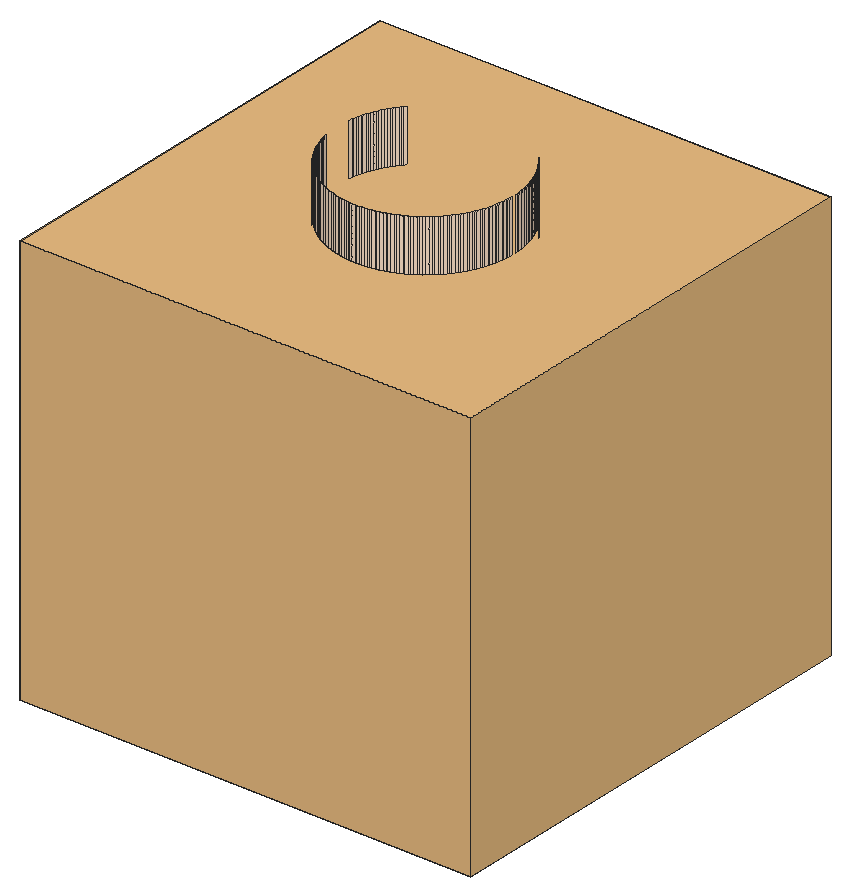
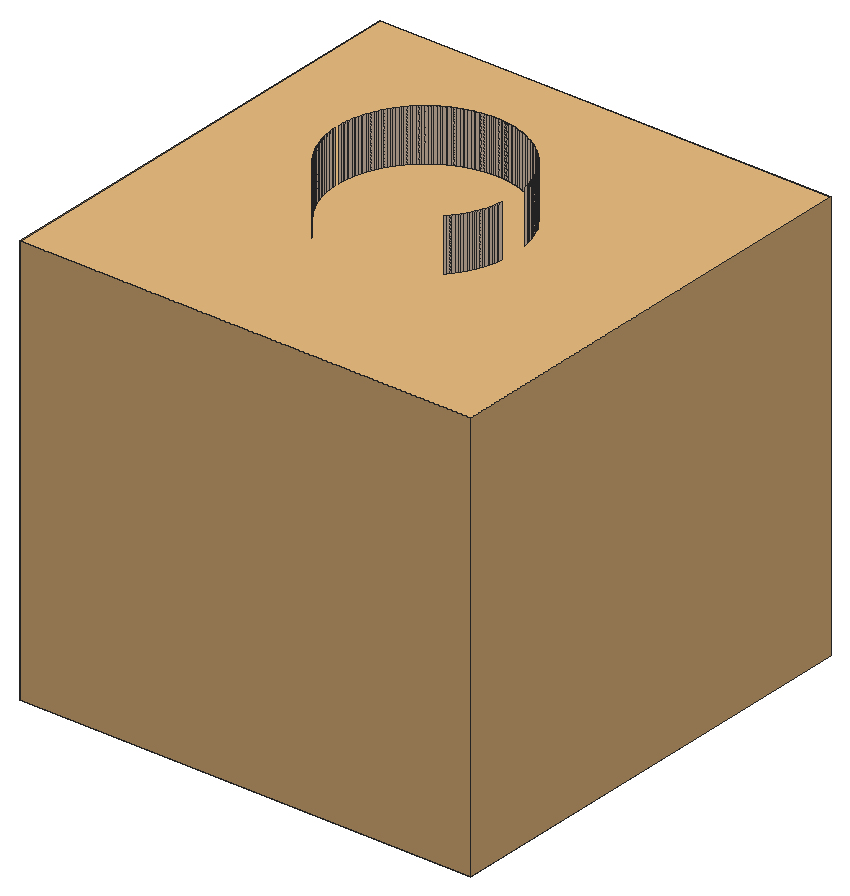
# SketchUp Ruby script. Lengths in inches.
U = 1.inch
M = Sketchup.active_model
def pt(a) = Geom::Point3d.new(a.map { |v| v * U })
def face(e, loops, mat)
  f = e.add_face(loops[0].map { |a| pt(a) })
  loops[1..].each { |l| e.add_face(l.map { |a| pt(a) }).erase! }
  f.material = f.back_material = mat if mat
  f
end
# faces: each face lists its corners as indices into pts; further lists are holes
def faces(e, pts, list, mat = nil) = list.each { |f| face(e, (f[0].is_a?(Array) ? f : [f]).map { |l| l.map { |i| pts[i] } }, mat) }
# xy, xz, yz: faces in a plane at the given z, y or x. An outline is a flat list of corners, or four numbers for a rectangle; further outlines are holes
def ring(l) = l.size == 4 ? [[l[0], l[1]], [l[2], l[1]], [l[2], l[3]], [l[0], l[3]]] : l.each_slice(2).to_a
def flat(e, list, mat, &to3) = list.each { |f| face(e, (f[0].is_a?(Array) ? f : [f]).map { |l| ring(l).map { |u, v| to3.(u, v) } }, mat) }
def xy(e, z, list, mat = nil) = flat(e, list, mat) { |x, y| [x, y, z] }
def xz(e, y, list, mat = nil) = flat(e, list, mat) { |x, z| [x, y, z] }
def yz(e, x, list, mat = nil) = flat(e, list, mat) { |y, z| [x, y, z] }
def lines(e, pts, list) = list.each { |a, b| e.add_line(pt(pts[a]), pt(pts[b])) }
# prism: a flat outline (further loops are holes) pulled along v
def prism(e, loops, v, mat = nil)
  f = face(e, loops, mat); d = Geom::Vector3d.new(v.map { |x| x * U })
  f.pushpull(f.normal.samedirection?(d) ? d.length : -d.length)
end
def box(e, o, s, mat = nil) = prism(e, [[o, [o[0] + s[0], o[1], o[2]], [o[0] + s[0], o[1] + s[1], o[2]], [o[0], o[1] + s[1], o[2]]]], [0, 0, s[2]], mat)
def at(x, y, z, deg = 0) = Geom::Transformation.translation(pt([x, y, z])) * Geom::Transformation.rotation(ORIGIN, Z_AXIS, deg.degrees)
def axes(o, x, y, z) = Geom::Transformation.new([*x, 0, *y, 0, *z, 0, *pt(o).to_a, 1])
def part(name) = M.definitions.add(name)
# library, detail: a bought-in or finely detailed component or shape, given as its bounding box
def library(name, o, s) = part(name).tap { |d| box(d.entities, o, s) }
def detail(e, o, s) = box(e.add_group.entities, o, s)
def put(e, d, t, mat = nil) = e.add_instance(d, t).tap { |i| i.material = mat if mat }
def group(e, t, mat = nil) = e.add_group.tap { |g| g.transformation = t; g.material = mat if mat }.entities
root = M.entities
M.materials.add("1122 AP 7994 PEACH ROSE").color = [254, 227, 201]
c1 = library("9",[-5.85,-5.85,-13.96],[15.28,15.28,13.96])
xz(root,174,[[52.82,278.82,52.9,281.82],[52.9,278.82,52.98,281.82],[52.98,278.82,53.06,281.82],[53.06,278.82,53.14,281.82]],"1122 AP 7994 PEACH ROSE")
yz(root,55.96,[[176.61,278.82,176.6875,281.82],[177.3125,278.82,177.39,281.82]],"1122 AP 7994 PEACH ROSE")
yz(root,55.98,[[176.84,278.82,176.92,281.82],[177.08,278.82,177.16,281.82]],"1122 AP 7994 PEACH ROSE")
p = [[52.51,174.04,278.82],[52.43,174.05,278.82],[52.43,174.05,281.82],[52.51,174.04,281.82],[52.59,174.03,278.82],[52.59,174.03,281.82],
  [52.67,174.02,278.82],[52.67,174.02,281.82],[52.75,174.01,278.82],[52.75,174.01,281.82],[52.82,174,278.82],[52.82,174,281.82],
  [53.22,174.01,278.82],[53.14,174,278.82],[53.14,174,281.82],[53.22,174.01,281.82],[53.29,174.02,278.82],[53.29,174.02,281.82],
  [53.37,174.03,278.82],[53.37,174.03,281.82],[53.45,174.04,278.82],[53.45,174.04,281.82],[53.53,174.05,278.82],[53.53,174.05,281.82],
  [52.05,174.15,278.82],[51.98,174.17,278.82],[51.98,174.17,281.82],[52.05,174.15,281.82],[52.13,174.125,278.82],[52.13,174.125,281.82],
  [52.2,174.1,278.82],[52.2,174.1,281.82],[52.28,174.08,278.82],[52.28,174.08,281.82],[52.36,174.07,278.82],[52.36,174.07,281.82],
  [53.6,174.07,278.82],[53.6,174.07,281.82],[53.68,174.08,278.82],[53.68,174.08,281.82],[53.76,174.1,278.82],[53.76,174.1,281.82],
  [53.83,174.125,278.82],[53.83,174.125,281.82],[53.91,174.15,278.82],[53.91,174.15,281.82],[53.98,174.17,278.82],[53.98,174.17,281.82],
  [51.83,174.23,278.82],[51.76,174.26,278.82],[51.76,174.26,281.82],[51.83,174.23,281.82],[51.91,174.2,278.82],[51.91,174.2,281.82],
  [54.06,174.2,278.82],[54.06,174.2,281.82],[54.13,174.23,278.82],[54.13,174.23,281.82],[54.2,174.26,278.82],[54.2,174.26,281.82],
  [51.62,174.33,278.82],[51.55,174.36,278.82],[51.55,174.36,281.82],[51.62,174.33,281.82],[51.6875,174.29,278.82],[51.6875,174.29,281.82],
  [54.27,174.29,278.82],[54.27,174.29,281.82],[54.34,174.33,278.82],[54.34,174.33,281.82],[54.41,174.36,278.82],[54.41,174.36,281.82],
  [51.41,174.44,278.82],[51.35,174.48,278.82],[51.35,174.48,281.82],[51.41,174.44,281.82],[51.48,174.4,278.82],[51.48,174.4,281.82],
  [54.48,174.4,278.82],[54.48,174.4,281.82],[54.55,174.44,278.82],[54.55,174.44,281.82],[54.61,174.48,278.82],[54.61,174.48,281.82],
  [51.28,174.53,278.82],[51.22,174.57,278.82],[51.22,174.57,281.82],[51.28,174.53,281.82],[54.68,174.53,278.82],[54.68,174.53,281.82],
  [54.74,174.57,278.82],[54.74,174.57,281.82],[51.15,174.62,278.82],[51.09,174.67,278.82],[51.09,174.67,281.82],[51.15,174.62,281.82],
  [54.81,174.62,278.82],[54.81,174.62,281.82],[54.87,174.67,278.82],[54.87,174.67,281.82],[51.03,174.72,278.82],[50.97,174.77,278.82],
  [50.97,174.77,281.82],[51.03,174.72,281.82],[54.93,174.72,278.82],[54.93,174.72,281.82],[54.99,174.77,278.82],[54.99,174.77,281.82],
  [50.92,174.82,278.82],[50.86,174.88,278.82],[50.86,174.88,281.82],[50.92,174.82,281.82],[55.05,174.82,278.82],[55.05,174.82,281.82],
  [55.1,174.88,278.82],[55.1,174.88,281.82],[50.8,174.93,278.82],[50.75,174.99,278.82],[50.75,174.99,281.82],[50.8,174.93,281.82],
  [55.16,174.93,278.82],[55.16,174.93,281.82],[55.21,174.99,278.82],[55.21,174.99,281.82],[50.7,175.05,278.82],[50.7,175.05,281.82],
  [55.26,175.05,278.82],[55.26,175.05,281.82],[50.65,175.11,278.82],[50.6,175.17,278.82],[50.6,175.17,281.82],[50.65,175.11,281.82],
  [55.3125,175.11,278.82],[55.3125,175.11,281.82],[55.36,175.17,278.82],[55.36,175.17,281.82],[50.55,175.24,278.82],[50.51,175.3,278.82],
  [50.51,175.3,281.82],[50.55,175.24,281.82],[55.41,175.24,278.82],[55.41,175.24,281.82],[55.45,175.3,278.82],[55.45,175.3,281.82],
  [50.46,175.37,278.82],[50.46,175.37,281.82],[55.5,175.37,278.82],[55.5,175.37,281.82],[50.42,175.43,278.82],[50.38,175.5,278.82],
  [50.38,175.5,281.82],[50.42,175.43,281.82],[55.54,175.43,278.82],[55.54,175.43,281.82],[55.58,175.5,278.82],[55.58,175.5,281.82],
  [50.34,175.57,278.82],[50.34,175.57,281.82],[55.62,175.57,278.82],[55.62,175.57,281.82],[50.31,175.64,278.82],[50.27,175.71,278.82],
  [50.27,175.71,281.82],[50.31,175.64,281.82],[55.65,175.64,278.82],[55.65,175.64,281.82],[55.6875,175.71,278.82],[55.6875,175.71,281.82],
  [50.24,175.78,278.82],[50.24,175.78,281.82],[55.72,175.78,278.82],[55.72,175.78,281.82],[50.21,175.85,278.82],[50.21,175.85,281.82],
  [55.75,175.85,278.82],[55.75,175.85,281.82],[50.18,175.92,278.82],[50.15,176,278.82],[50.15,176,281.82],[50.18,175.92,281.82],
  [55.78,175.92,278.82],[55.78,175.92,281.82],[55.81,176,278.82],[55.81,176,281.82],[50.13,176.07,278.82],[50.13,176.07,281.82],
  [55.83,176.07,278.82],[55.83,176.07,281.82],[50.1,176.15,278.82],[50.08,176.22,278.82],[50.08,176.22,281.82],[50.1,176.15,281.82],
  [55.86,176.15,278.82],[55.86,176.15,281.82],[55.88,176.22,278.82],[55.88,176.22,281.82],[50.0625,176.3,278.82],[50.0625,176.3,281.82],
  [55.9,176.3,278.82],[55.9,176.3,281.82],[50.05,176.375,278.82],[50.05,176.375,281.82],[55.92,176.375,278.82],[55.92,176.375,281.82],
  [50.03,176.45,278.82],[50.03,176.45,281.82],[55.93,176.45,278.82],[55.93,176.45,281.82],[55.94,176.53,278.82],[55.94,176.53,281.82],
  [55.96,176.61,278.82],[55.96,176.61,281.82],[55.97,176.76,278.82],[55.96,176.6875,278.82],[55.96,176.6875,281.82],[55.97,176.76,281.82],
  [55.98,176.84,278.82],[55.98,176.84,281.82],[55.96,177.3125,278.82],[55.97,177.24,278.82],[55.97,177.24,281.82],[55.96,177.3125,281.82],
  [55.98,177.16,278.82],[55.98,177.16,281.82],[55.94,177.47,278.82],[55.96,177.39,278.82],[55.96,177.39,281.82],[55.94,177.47,281.82],
  [50.02,177.47,278.82],[50.03,177.55,278.82],[50.03,177.55,281.82],[50.02,177.47,281.82],[50.05,177.625,278.82],[50.05,177.625,281.82],
  [55.92,177.625,278.82],[55.93,177.55,278.82],[55.93,177.55,281.82],[55.92,177.625,281.82],[50.0625,177.7,278.82],[50.0625,177.7,281.82],
  [55.9,177.7,278.82],[55.9,177.7,281.82],[50.08,177.78,278.82],[50.08,177.78,281.82],[55.88,177.78,278.82],[55.88,177.78,281.82],
  [50.1,177.85,278.82],[50.1,177.85,281.82],[55.86,177.85,278.82],[55.86,177.85,281.82],[50.13,177.93,278.82],[50.13,177.93,281.82],
  [50.15,178,278.82],[50.15,178,281.82],[55.81,178,278.82],[55.83,177.93,278.82],[55.83,177.93,281.82],[55.81,178,281.82],
  [50.18,178.08,278.82],[50.18,178.08,281.82],[55.78,178.08,278.82],[55.78,178.08,281.82],[50.21,178.15,278.82],[50.21,178.15,281.82],
  [50.24,178.22,278.82],[50.24,178.22,281.82],[55.72,178.22,278.82],[55.75,178.15,278.82],[55.75,178.15,281.82],[55.72,178.22,281.82],
  [50.27,178.29,278.82],[50.27,178.29,281.82],[55.6875,178.29,278.82],[55.6875,178.29,281.82],[50.31,178.36,278.82],[50.31,178.36,281.82],
  [55.65,178.36,278.82],[55.65,178.36,281.82],[50.34,178.43,278.82],[50.34,178.43,281.82],[50.38,178.5,278.82],[50.38,178.5,281.82],
  [55.58,178.5,278.82],[55.62,178.43,278.82],[55.62,178.43,281.82],[55.58,178.5,281.82],[50.42,178.57,278.82],[50.42,178.57,281.82],
  [55.54,178.57,278.82],[55.54,178.57,281.82],[50.46,178.63,278.82],[50.46,178.63,281.82],[50.51,178.7,278.82],[50.51,178.7,281.82],
  [55.45,178.7,278.82],[55.5,178.63,278.82],[55.5,178.63,281.82],[55.45,178.7,281.82],[50.55,178.76,278.82],[50.55,178.76,281.82],
  [55.41,178.76,278.82],[55.41,178.76,281.82],[50.6,178.83,278.82],[50.6,178.83,281.82],[50.65,178.89,278.82],[50.65,178.89,281.82],
  [55.3125,178.89,278.82],[55.36,178.83,278.82],[55.36,178.83,281.82],[55.3125,178.89,281.82],[50.7,178.95,278.82],[50.7,178.95,281.82],
  [50.75,179.01,278.82],[50.75,179.01,281.82],[55.21,179.01,278.82],[55.26,178.95,278.82],[55.26,178.95,281.82],[55.21,179.01,281.82]]
faces(root,p,[[0,1,2,3],[4,0,3,5],[6,4,5,7],[8,6,7,9],[10,8,9,11],[12,13,14,15],[16,12,15,17],[18,16,17,19],
  [20,18,19,21],[22,20,21,23],[24,25,26,27],[28,24,27,29],[30,28,29,31],[32,30,31,33],[34,32,33,35],[1,34,35,2],
  [36,22,23,37],[38,36,37,39],[40,38,39,41],[42,40,41,43],[44,42,43,45],[46,44,45,47],[48,49,50,51],[52,48,51,53],
  [25,52,53,26],[54,46,47,55],[56,54,55,57],[58,56,57,59],[60,61,62,63],[64,60,63,65],[49,64,65,50],[66,58,59,67],
  [68,66,67,69],[70,68,69,71],[72,73,74,75],[76,72,75,77],[61,76,77,62],[78,70,71,79],[80,78,79,81],[82,80,81,83],
  [84,85,86,87],[73,84,87,74],[88,82,83,89],[90,88,89,91],[92,93,94,95],[85,92,95,86],[96,90,91,97],[98,96,97,99],
  [100,101,102,103],[93,100,103,94],[104,98,99,105],[106,104,105,107],[108,109,110,111],[101,108,111,102],[112,106,107,113],[114,112,113,115],
  [116,117,118,119],[109,116,119,110],[120,114,115,121],[122,120,121,123],[117,124,125,118],[126,122,123,127],[128,129,130,131],[124,128,131,125],
  [132,126,127,133],[134,132,133,135],[136,137,138,139],[129,136,139,130],[140,134,135,141],[142,140,141,143],[137,144,145,138],[146,142,143,147],
  [148,149,150,151],[144,148,151,145],[152,146,147,153],[154,152,153,155],[149,156,157,150],[158,154,155,159],[160,161,162,163],[156,160,163,157],
  [164,158,159,165],[166,164,165,167],[161,168,169,162],[170,166,167,171],[168,172,173,169],[174,170,171,175],[176,177,178,179],[172,176,179,173],
  [180,174,175,181],[182,180,181,183],[177,184,185,178],[186,182,183,187],[188,189,190,191],[184,188,191,185],[192,186,187,193],[194,192,193,195],
  [189,196,197,190],[198,194,195,199],[196,200,201,197],[202,198,199,203],[200,204,205,201],[206,202,203,207],[208,206,207,209],[210,208,209,211],
  [212,213,214,215],[216,212,215,217],[218,219,220,221],[219,222,223,220],[224,225,226,227],[228,229,230,231],[229,232,233,230],[234,235,236,237],
  [235,224,227,236],[232,238,239,233],[240,234,237,241],[238,242,243,239],[244,240,241,245],[242,246,247,243],[248,244,245,249],[246,250,251,247],
  [250,252,253,251],[254,255,256,257],[255,248,249,256],[252,258,259,253],[260,254,257,261],[258,262,263,259],[262,264,265,263],[266,267,268,269],
  [267,260,261,268],[264,270,271,265],[272,266,269,273],[270,274,275,271],[276,272,273,277],[274,278,279,275],[278,280,281,279],[282,283,284,285],
  [283,276,277,284],[280,286,287,281],[288,282,285,289],[286,290,291,287],[290,292,293,291],[294,295,296,297],[295,288,289,296],[292,298,299,293],
  [300,294,297,301],[298,302,303,299],[302,304,305,303],[306,307,308,309],[307,300,301,308],[304,310,311,305],[310,312,313,311],[314,315,316,317],
  [315,306,309,316]],"1122 AP 7994 PEACH ROSE")
put(root,c1,at(51.19,175.21,280.07))
